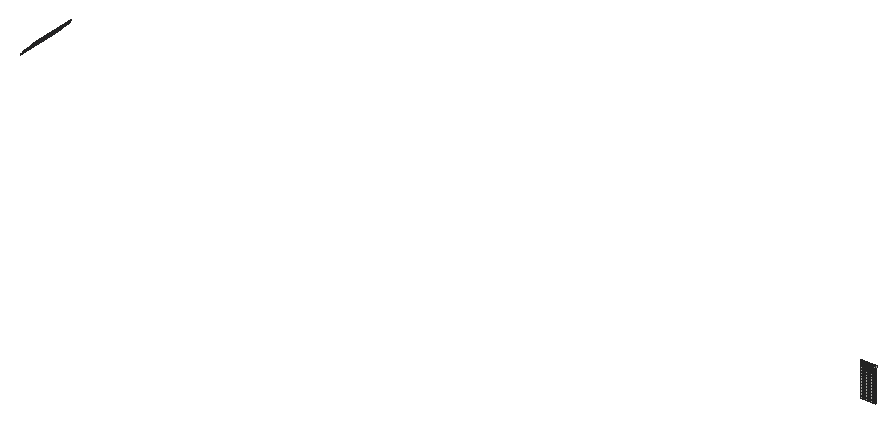
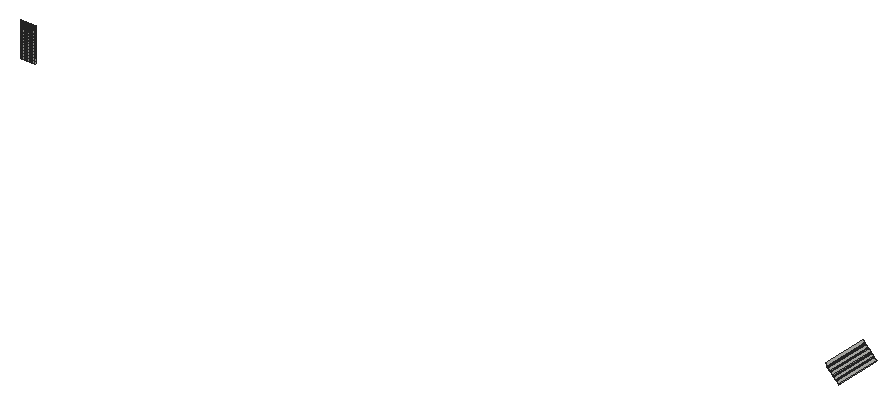
# SketchUp Ruby script. Lengths in inches.
U = 1.inch
M = Sketchup.active_model
def pt(a) = Geom::Point3d.new(a.map { |v| v * U })
def face(e, loops, mat)
  f = e.add_face(loops[0].map { |a| pt(a) })
  loops[1..].each { |l| e.add_face(l.map { |a| pt(a) }).erase! }
  f.material = f.back_material = mat if mat
  f
end
# faces: each face lists its corners as indices into pts; further lists are holes
def faces(e, pts, list, mat = nil) = list.each { |f| face(e, (f[0].is_a?(Array) ? f : [f]).map { |l| l.map { |i| pts[i] } }, mat) }
# xy, xz, yz: faces in a plane at the given z, y or x. An outline is a flat list of corners, or four numbers for a rectangle; further outlines are holes
def ring(l) = l.size == 4 ? [[l[0], l[1]], [l[2], l[1]], [l[2], l[3]], [l[0], l[3]]] : l.each_slice(2).to_a
def flat(e, list, mat, &to3) = list.each { |f| face(e, (f[0].is_a?(Array) ? f : [f]).map { |l| ring(l).map { |u, v| to3.(u, v) } }, mat) }
def xy(e, z, list, mat = nil) = flat(e, list, mat) { |x, y| [x, y, z] }
def xz(e, y, list, mat = nil) = flat(e, list, mat) { |x, z| [x, y, z] }
def yz(e, x, list, mat = nil) = flat(e, list, mat) { |y, z| [x, y, z] }
def lines(e, pts, list) = list.each { |a, b| e.add_line(pt(pts[a]), pt(pts[b])) }
# prism: a flat outline (further loops are holes) pulled along v
def prism(e, loops, v, mat = nil)
  f = face(e, loops, mat); d = Geom::Vector3d.new(v.map { |x| x * U })
  f.pushpull(f.normal.samedirection?(d) ? d.length : -d.length)
end
def box(e, o, s, mat = nil) = prism(e, [[o, [o[0] + s[0], o[1], o[2]], [o[0] + s[0], o[1] + s[1], o[2]], [o[0], o[1] + s[1], o[2]]]], [0, 0, s[2]], mat)
def at(x, y, z, deg = 0) = Geom::Transformation.translation(pt([x, y, z])) * Geom::Transformation.rotation(ORIGIN, Z_AXIS, deg.degrees)
def axes(o, x, y, z) = Geom::Transformation.new([*x, 0, *y, 0, *z, 0, *pt(o).to_a, 1])
def part(name) = M.definitions.add(name)
# library, detail: a bought-in or finely detailed component or shape, given as its bounding box
def library(name, o, s) = part(name).tap { |d| box(d.entities, o, s) }
def detail(e, o, s) = box(e.add_group.entities, o, s)
def put(e, d, t, mat = nil) = e.add_instance(d, t).tap { |i| i.material = mat if mat }
def group(e, t, mat = nil) = e.add_group.tap { |g| g.transformation = t; g.material = mat if mat }.entities
root = M.entities
M.materials.add("[Color M06]").color = [79, 71, 84]
xy(root,265.77,[[2255.22,480.14,2257.54,480.77],[2258.14,480.14,2260.45,480.77],[2261.05,480.14,2263.36,480.77],[2263.96,480.14,2266.27,480.77],[2266.87,480.14,2269.19,480.77],
  [2269.78,480.14,2272.1,480.77]])
xy(root,268.09,[[2255.22,480.14,2257.54,480.77],[2258.14,480.14,2260.45,480.77],[2261.05,480.14,2263.36,480.77],[2263.96,480.14,2266.27,480.77],[2266.87,480.14,2269.19,480.77],
  [2269.78,480.14,2272.1,480.77]])
xy(root,268.82,[[2255.25,480.14,2257.57,480.77],[2258.17,480.14,2260.48,480.77],[2261.08,480.14,2263.39,480.77],[2263.99,480.14,2266.3,480.77],[2266.9,480.14,2269.21,480.77],
  [2269.8125,480.14,2272.125,480.77]])
xy(root,271.13,[[2255.25,480.14,2257.57,480.77],[2258.17,480.14,2260.48,480.77],[2261.08,480.14,2263.39,480.77],[2263.99,480.14,2266.3,480.77],[2266.9,480.14,2269.21,480.77],
  [2269.8125,480.14,2272.125,480.77]])
xy(root,271.86,[[2255.28,480.14,2257.6,480.77],[2258.19,480.14,2260.51,480.77],[2261.11,480.14,2263.42,480.77],[2264.02,480.14,2266.33,480.77],[2266.93,480.14,2269.24,480.77],
  [2269.84,480.14,2272.16,480.77]])
xy(root,274.17,[[2255.28,480.14,2257.6,480.77],[2258.19,480.14,2260.51,480.77],[2261.11,480.14,2263.42,480.77],[2264.02,480.14,2266.33,480.77],[2266.93,480.14,2269.24,480.77],
  [2269.84,480.14,2272.16,480.77]])
xy(root,274.91,[[2255.3125,480.14,2257.625,480.77],[2258.22,480.14,2260.54,480.77],[2261.14,480.14,2263.45,480.77],[2264.05,480.14,2266.36,480.77],[2266.96,480.14,2269.27,480.77],
  [2269.87,480.14,2272.18,480.77]])
xy(root,277.22,[[2255.3125,480.14,2257.625,480.77],[2258.22,480.14,2260.54,480.77],[2261.14,480.14,2263.45,480.77],[2264.05,480.14,2266.36,480.77],[2266.96,480.14,2269.27,480.77],
  [2269.87,480.14,2272.18,480.77]])
xy(root,277.95,[[2255.34,480.14,2257.65,480.77],[2258.25,480.14,2260.57,480.77],[2261.16,480.14,2263.48,480.77],[2264.08,480.14,2266.39,480.77],[2266.99,480.14,2269.3,480.77],
  [2269.9,480.14,2272.21,480.77]])
xy(root,280.26,[[2255.34,480.14,2257.65,480.77],[2258.25,480.14,2260.57,480.77],[2261.16,480.14,2263.48,480.77],[2264.08,480.14,2266.39,480.77],[2266.99,480.14,2269.3,480.77],
  [2269.9,480.14,2272.21,480.77]])
xy(root,281,[[2255.37,480.14,2257.68,480.77],[2258.28,480.14,2260.59,480.77],[2261.19,480.14,2263.51,480.77],[2264.11,480.14,2266.42,480.77],[2267.02,480.14,2269.33,480.77],
  [2269.93,480.14,2272.24,480.77]])
xy(root,283.31,[[2255.37,480.14,2257.68,480.77],[2258.28,480.14,2260.59,480.77],[2261.19,480.14,2263.51,480.77],[2264.11,480.14,2266.42,480.77],[2267.02,480.14,2269.33,480.77],
  [2269.93,480.14,2272.24,480.77]])
xy(root,284.04,[[2255.4,480.14,2257.71,480.77],[2258.3125,480.14,2260.625,480.77],[2261.22,480.14,2263.54,480.77],[2264.13,480.14,2266.45,480.77],[2267.05,480.14,2269.36,480.77],
  [2269.96,480.14,2272.27,480.77]])
xy(root,286.35,[[2255.4,480.14,2257.71,480.77],[2258.3125,480.14,2260.625,480.77],[2261.22,480.14,2263.54,480.77],[2264.13,480.14,2266.45,480.77],[2267.05,480.14,2269.36,480.77],
  [2269.96,480.14,2272.27,480.77]])
xy(root,287.09,[[2255.43,480.14,2257.74,480.77],[2258.34,480.14,2260.65,480.77],[2261.25,480.14,2263.5625,480.77],[2264.16,480.14,2266.48,480.77],[2267.08,480.14,2269.39,480.77],
  [2269.99,480.14,2272.3,480.77]])
xy(root,289.4,[[2255.43,480.14,2257.74,480.77],[2258.34,480.14,2260.65,480.77],[2261.25,480.14,2263.5625,480.77],[2264.16,480.14,2266.48,480.77],[2267.08,480.14,2269.39,480.77],
  [2269.99,480.14,2272.3,480.77]])
xy(root,290.13,[[2255.46,480.14,2257.77,480.77],[2258.37,480.14,2260.68,480.77],[2261.28,480.14,2263.59,480.77],[2264.19,480.14,2266.51,480.77],[2267.1,480.14,2269.42,480.77],
  [2270.02,480.14,2272.33,480.77]])
xy(root,292.44,[[2255.46,480.14,2257.77,480.77],[2258.37,480.14,2260.68,480.77],[2261.28,480.14,2263.59,480.77],[2264.19,480.14,2266.51,480.77],[2267.1,480.14,2269.42,480.77],
  [2270.02,480.14,2272.33,480.77]])
xy(root,293.18,[[2255.49,480.14,2257.8,480.77],[2258.4,480.14,2260.71,480.77],[2261.31,480.14,2263.62,480.77],[2264.22,480.14,2266.53,480.77],[2267.13,480.14,2269.45,480.77],
  [2270.05,480.14,2272.36,480.77]])
xy(root,295.49,[[2255.49,480.14,2257.8,480.77],[2258.4,480.14,2260.71,480.77],[2261.31,480.14,2263.62,480.77],[2264.22,480.14,2266.53,480.77],[2267.13,480.14,2269.45,480.77],
  [2270.05,480.14,2272.36,480.77]])
xy(root,296.22,[[2255.51,480.14,2257.83,480.77],[2258.43,480.14,2260.74,480.77],[2261.34,480.14,2263.65,480.77],[2264.25,480.14,2266.5625,480.77],[2267.16,480.14,2269.48,480.77],
  [2270.07,480.14,2272.39,480.77]])
xy(root,298.53,[[2255.51,480.14,2257.83,480.77],[2258.43,480.14,2260.74,480.77],[2261.34,480.14,2263.65,480.77],[2264.25,480.14,2266.5625,480.77],[2267.16,480.14,2269.48,480.77],
  [2270.07,480.14,2272.39,480.77]])
xy(root,299.27,[[2255.54,480.14,2257.86,480.77],[2258.46,480.14,2260.77,480.77],[2261.37,480.14,2263.68,480.77],[2264.28,480.14,2266.59,480.77],[2267.19,480.14,2269.5,480.77],
  [2270.1,480.14,2272.42,480.77]])
xy(root,301.58,[[2255.54,480.14,2257.86,480.77],[2258.46,480.14,2260.77,480.77],[2261.37,480.14,2263.68,480.77],[2264.28,480.14,2266.59,480.77],[2267.19,480.14,2269.5,480.77],
  [2270.1,480.14,2272.42,480.77]])
xy(root,302.31,[[2255.57,480.14,2257.89,480.77],[2258.48,480.14,2260.8,480.77],[2261.4,480.14,2263.71,480.77],[2264.31,480.14,2266.62,480.77],[2267.22,480.14,2269.53,480.77],
  [2270.13,480.14,2272.45,480.77]])
xy(root,304.62,[[2255.57,480.14,2257.89,480.77],[2258.48,480.14,2260.8,480.77],[2261.4,480.14,2263.71,480.77],[2264.31,480.14,2266.62,480.77],[2267.22,480.14,2269.53,480.77],
  [2270.13,480.14,2272.45,480.77]])
yz(root,2254.68,[[480.14,271.86,480.77,274.17]])
yz(root,2254.71,[[480.14,274.91,480.77,277.22]])
yz(root,2254.74,[[480.14,277.95,480.77,280.26]])
yz(root,2254.77,[[480.14,281,480.77,283.31]])
yz(root,2254.8,[[480.14,284.04,480.77,286.35]])
yz(root,2254.83,[[480.14,287.09,480.77,289.4]])
yz(root,2254.86,[[480.14,290.13,480.77,292.44]])
yz(root,2254.89,[[480.14,293.18,480.77,295.49]])
yz(root,2254.91,[[480.14,296.22,480.77,298.53]])
yz(root,2254.94,[[480.14,299.27,480.77,301.58]])
yz(root,2254.97,[[480.14,302.31,480.77,304.62]])
yz(root,2255.22,[[480.14,265.77,480.77,268.09]])
yz(root,2255.25,[[480.14,268.82,480.77,271.13]])
yz(root,2255.28,[[480.14,271.86,480.77,274.17]])
yz(root,2255.3125,[[480.14,274.91,480.77,277.22]])
yz(root,2255.34,[[480.14,277.95,480.77,280.26]])
yz(root,2255.37,[[480.14,281,480.77,283.31]])
yz(root,2255.4,[[480.14,284.04,480.77,286.35]])
yz(root,2255.43,[[480.14,287.09,480.77,289.4]])
yz(root,2255.46,[[480.14,290.13,480.77,292.44]])
yz(root,2255.49,[[480.14,293.18,480.77,295.49]])
yz(root,2255.51,[[480.14,296.22,480.77,298.53]])
yz(root,2255.54,[[480.14,299.27,480.77,301.58]])
yz(root,2255.57,[[480.14,302.31,480.77,304.62]])
yz(root,2257.54,[[480.14,265.77,480.77,268.09]])
yz(root,2257.57,[[480.14,268.82,480.77,271.13]])
yz(root,2257.6,[[480.14,271.86,480.77,274.17]])
yz(root,2257.625,[[480.14,274.91,480.77,277.22]])
yz(root,2257.65,[[480.14,277.95,480.77,280.26]])
yz(root,2257.68,[[480.14,281,480.77,283.31]])
yz(root,2257.71,[[480.14,284.04,480.77,286.35]])
yz(root,2257.74,[[480.14,287.09,480.77,289.4]])
yz(root,2257.77,[[480.14,290.13,480.77,292.44]])
yz(root,2257.8,[[480.14,293.18,480.77,295.49]])
yz(root,2257.83,[[480.14,296.22,480.77,298.53]])
yz(root,2257.86,[[480.14,299.27,480.77,301.58]])
yz(root,2257.89,[[480.14,302.31,480.77,304.62]])
yz(root,2258.14,[[480.14,265.77,480.77,268.09]])
yz(root,2258.17,[[480.14,268.82,480.77,271.13]])
yz(root,2258.19,[[480.14,271.86,480.77,274.17]])
yz(root,2258.22,[[480.14,274.91,480.77,277.22]])
yz(root,2258.25,[[480.14,277.95,480.77,280.26]])
yz(root,2258.28,[[480.14,281,480.77,283.31]])
yz(root,2258.3125,[[480.14,284.04,480.77,286.35]])
yz(root,2258.34,[[480.14,287.09,480.77,289.4]])
yz(root,2258.37,[[480.14,290.13,480.77,292.44]])
yz(root,2258.4,[[480.14,293.18,480.77,295.49]])
yz(root,2258.43,[[480.14,296.22,480.77,298.53]])
yz(root,2258.46,[[480.14,299.27,480.77,301.58]])
yz(root,2258.48,[[480.14,302.31,480.77,304.62]])
yz(root,2260.45,[[480.14,265.77,480.77,268.09]])
yz(root,2260.48,[[480.14,268.82,480.77,271.13]])
yz(root,2260.51,[[480.14,271.86,480.77,274.17]])
yz(root,2260.54,[[480.14,274.91,480.77,277.22]])
yz(root,2260.57,[[480.14,277.95,480.77,280.26]])
yz(root,2260.59,[[480.14,281,480.77,283.31]])
yz(root,2260.625,[[480.14,284.04,480.77,286.35]])
yz(root,2260.65,[[480.14,287.09,480.77,289.4]])
yz(root,2260.68,[[480.14,290.13,480.77,292.44]])
yz(root,2260.71,[[480.14,293.18,480.77,295.49]])
yz(root,2260.74,[[480.14,296.22,480.77,298.53]])
yz(root,2260.77,[[480.14,299.27,480.77,301.58]])
yz(root,2260.8,[[480.14,302.31,480.77,304.62]])
yz(root,2261.05,[[480.14,265.77,480.77,268.09]])
yz(root,2261.08,[[480.14,268.82,480.77,271.13]])
yz(root,2261.11,[[480.14,271.86,480.77,274.17]])
yz(root,2261.14,[[480.14,274.91,480.77,277.22]])
yz(root,2261.16,[[480.14,277.95,480.77,280.26]])
yz(root,2261.19,[[480.14,281,480.77,283.31]])
yz(root,2261.22,[[480.14,284.04,480.77,286.35]])
yz(root,2261.25,[[480.14,287.09,480.77,289.4]])
yz(root,2261.28,[[480.14,290.13,480.77,292.44]])
yz(root,2261.31,[[480.14,293.18,480.77,295.49]])
yz(root,2261.34,[[480.14,296.22,480.77,298.53]])
yz(root,2261.37,[[480.14,299.27,480.77,301.58]])
yz(root,2261.4,[[480.14,302.31,480.77,304.62]])
yz(root,2263.36,[[480.14,265.77,480.77,268.09]])
yz(root,2263.39,[[480.14,268.82,480.77,271.13]])
yz(root,2263.42,[[480.14,271.86,480.77,274.17]])
yz(root,2263.45,[[480.14,274.91,480.77,277.22]])
yz(root,2263.48,[[480.14,277.95,480.77,280.26]])
yz(root,2263.51,[[480.14,281,480.77,283.31]])
yz(root,2263.54,[[480.14,284.04,480.77,286.35]])
yz(root,2263.5625,[[480.14,287.09,480.77,289.4]])
yz(root,2263.59,[[480.14,290.13,480.77,292.44]])
yz(root,2263.62,[[480.14,293.18,480.77,295.49]])
yz(root,2263.65,[[480.14,296.22,480.77,298.53]])
yz(root,2263.68,[[480.14,299.27,480.77,301.58]])
yz(root,2263.71,[[480.14,302.31,480.77,304.62]])
yz(root,2263.96,[[480.14,265.77,480.77,268.09]])
yz(root,2263.99,[[480.14,268.82,480.77,271.13]])
yz(root,2264.02,[[480.14,271.86,480.77,274.17]])
yz(root,2264.05,[[480.14,274.91,480.77,277.22]])
yz(root,2264.08,[[480.14,277.95,480.77,280.26]])
yz(root,2264.11,[[480.14,281,480.77,283.31]])
yz(root,2264.13,[[480.14,284.04,480.77,286.35]])
yz(root,2264.16,[[480.14,287.09,480.77,289.4]])
yz(root,2264.19,[[480.14,290.13,480.77,292.44]])
yz(root,2264.22,[[480.14,293.18,480.77,295.49]])
yz(root,2264.25,[[480.14,296.22,480.77,298.53]])
yz(root,2264.28,[[480.14,299.27,480.77,301.58]])
yz(root,2264.31,[[480.14,302.31,480.77,304.62]])
yz(root,2266.27,[[480.14,265.77,480.77,268.09]])
yz(root,2266.3,[[480.14,268.82,480.77,271.13]])
yz(root,2266.33,[[480.14,271.86,480.77,274.17]])
yz(root,2266.36,[[480.14,274.91,480.77,277.22]])
yz(root,2266.39,[[480.14,277.95,480.77,280.26]])
yz(root,2266.42,[[480.14,281,480.77,283.31]])
yz(root,2266.45,[[480.14,284.04,480.77,286.35]])
yz(root,2266.48,[[480.14,287.09,480.77,289.4]])
yz(root,2266.51,[[480.14,290.13,480.77,292.44]])
yz(root,2266.53,[[480.14,293.18,480.77,295.49]])
yz(root,2266.5625,[[480.14,296.22,480.77,298.53]])
yz(root,2266.59,[[480.14,299.27,480.77,301.58]])
yz(root,2266.62,[[480.14,302.31,480.77,304.62]])
yz(root,2266.87,[[480.14,265.77,480.77,268.09]])
yz(root,2266.9,[[480.14,268.82,480.77,271.13]])
yz(root,2266.93,[[480.14,271.86,480.77,274.17]])
yz(root,2266.96,[[480.14,274.91,480.77,277.22]])
yz(root,2266.99,[[480.14,277.95,480.77,280.26]])
yz(root,2267.02,[[480.14,281,480.77,283.31]])
yz(root,2267.05,[[480.14,284.04,480.77,286.35]])
yz(root,2267.08,[[480.14,287.09,480.77,289.4]])
yz(root,2267.1,[[480.14,290.13,480.77,292.44]])
yz(root,2267.13,[[480.14,293.18,480.77,295.49]])
yz(root,2267.16,[[480.14,296.22,480.77,298.53]])
yz(root,2267.19,[[480.14,299.27,480.77,301.58]])
yz(root,2267.22,[[480.14,302.31,480.77,304.62]])
yz(root,2269.19,[[480.14,265.77,480.77,268.09]])
yz(root,2269.21,[[480.14,268.82,480.77,271.13]])
yz(root,2269.24,[[480.14,271.86,480.77,274.17]])
yz(root,2269.27,[[480.14,274.91,480.77,277.22]])
yz(root,2269.3,[[480.14,277.95,480.77,280.26]])
yz(root,2269.33,[[480.14,281,480.77,283.31]])
yz(root,2269.36,[[480.14,284.04,480.77,286.35]])
yz(root,2269.39,[[480.14,287.09,480.77,289.4]])
yz(root,2269.42,[[480.14,290.13,480.77,292.44]])
yz(root,2269.45,[[480.14,293.18,480.77,295.49]])
yz(root,2269.48,[[480.14,296.22,480.77,298.53]])
yz(root,2269.5,[[480.14,299.27,480.77,301.58]])
yz(root,2269.53,[[480.14,302.31,480.77,304.62]])
yz(root,2269.78,[[480.14,265.77,480.77,268.09]])
yz(root,2269.8125,[[480.14,268.82,480.77,271.13]])
yz(root,2269.84,[[480.14,271.86,480.77,274.17]])
yz(root,2269.87,[[480.14,274.91,480.77,277.22]])
yz(root,2269.9,[[480.14,277.95,480.77,280.26]])
yz(root,2269.93,[[480.14,281,480.77,283.31]])
yz(root,2269.96,[[480.14,284.04,480.77,286.35]])
yz(root,2269.99,[[480.14,287.09,480.77,289.4]])
yz(root,2270.02,[[480.14,290.13,480.77,292.44]])
yz(root,2270.05,[[480.14,293.18,480.77,295.49]])
yz(root,2270.07,[[480.14,296.22,480.77,298.53]])
yz(root,2270.1,[[480.14,299.27,480.77,301.58]])
yz(root,2270.13,[[480.14,302.31,480.77,304.62]])
yz(root,2272.1,[[480.14,265.77,480.77,268.09]])
yz(root,2272.125,[[480.14,268.82,480.77,271.13]])
yz(root,2272.16,[[480.14,271.86,480.77,274.17]])
yz(root,2272.18,[[480.14,274.91,480.77,277.22]])
yz(root,2272.21,[[480.14,277.95,480.77,280.26]])
yz(root,2272.24,[[480.14,281,480.77,283.31]])
yz(root,2272.27,[[480.14,284.04,480.77,286.35]])
yz(root,2272.3,[[480.14,287.09,480.77,289.4]])
yz(root,2272.33,[[480.14,290.13,480.77,292.44]])
yz(root,2272.36,[[480.14,293.18,480.77,295.49]])
yz(root,2272.39,[[480.14,296.22,480.77,298.53]])
yz(root,2272.42,[[480.14,299.27,480.77,301.58]])
yz(root,2272.45,[[480.14,302.31,480.77,304.62]])
p = [[1288.59,467.1875,289.56],[1288.59,521.5625,289.56],[1289.04,521.5625,289.13],[1289.04,467.1875,289.13],[1291.46,521.5625,291.7],[1291.46,467.1875,291.7],
  [1291.01,521.5625,292.13],[1291.01,467.1875,292.13],[1291.88,521.5625,293.0625],[1291.88,467.1875,293.0625],[1292.34,521.5625,292.64],[1292.34,467.1875,292.64],
  [1294.76,521.5625,295.21],[1294.76,467.1875,295.21],[1294.3,521.5625,295.64],[1294.3,467.1875,295.64],[1295.18,521.5625,296.57],[1295.18,467.1875,296.57],
  [1295.64,521.5625,296.14],[1295.64,467.1875,296.14],[1298.06,521.5625,298.71],[1298.06,467.1875,298.71],[1297.6,521.5625,299.14],[1297.6,467.1875,299.14],
  [1298.48,521.5625,300.07],[1298.48,467.1875,300.07],[1298.9375,521.5625,299.64],[1298.9375,467.1875,299.64],[1301.36,521.5625,302.22],[1301.36,467.1875,302.22],
  [1300.9,521.5625,302.64],[1300.9,467.1875,302.64],[1301.78,521.5625,303.58],[1301.78,467.1875,303.58],[1302.23,521.5625,303.15],[1302.23,467.1875,303.15],
  [1301.55,467.1875,303.79],[1301.55,521.5625,303.79],[1304.2,521.5625,306.15],[1304.2,467.1875,306.15],[1303.97,521.5625,306.36],[1303.97,467.1875,306.36]]
faces(root,p,[[0,1,2,3],[6,1,0,7],[6,7,5,4],[9,8,10,11],[14,8,9,15],[14,15,13,12],[17,16,18,19],[22,16,17,23],
  [22,23,21,20],[25,24,26,27],[30,24,25,31],[30,31,29,28],[32,33,36,37],[38,32,33,39],[40,37,36,41]])
faces(root,p,[[2,4,5,3],[6,8,9,7],[10,12,13,11],[14,16,17,15],[18,20,21,19],[22,24,25,23],[26,28,29,27],[30,32,33,31],
  [33,32,34,35]],"[Color M06]")
